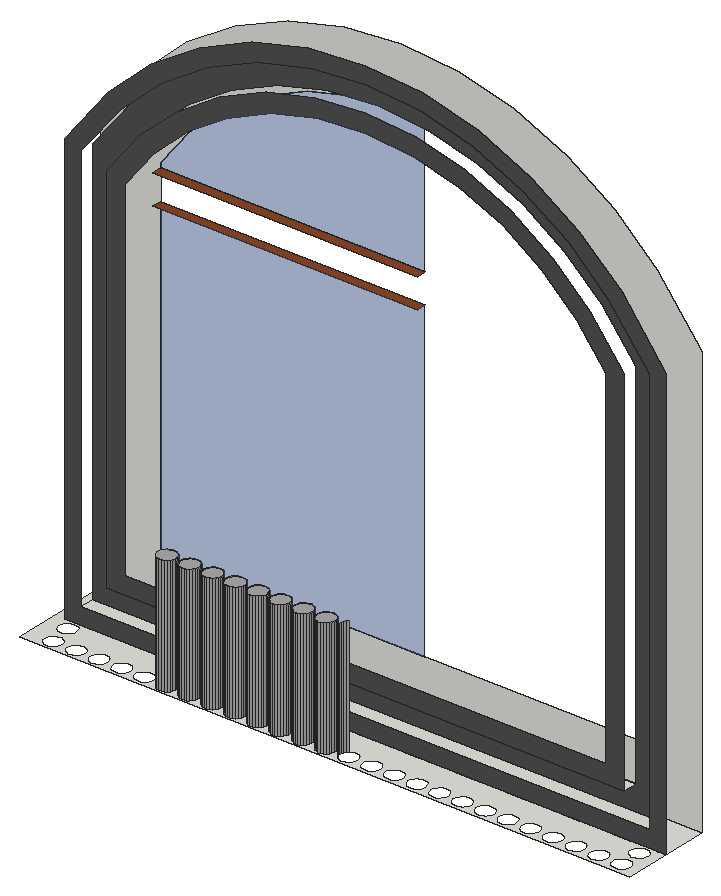
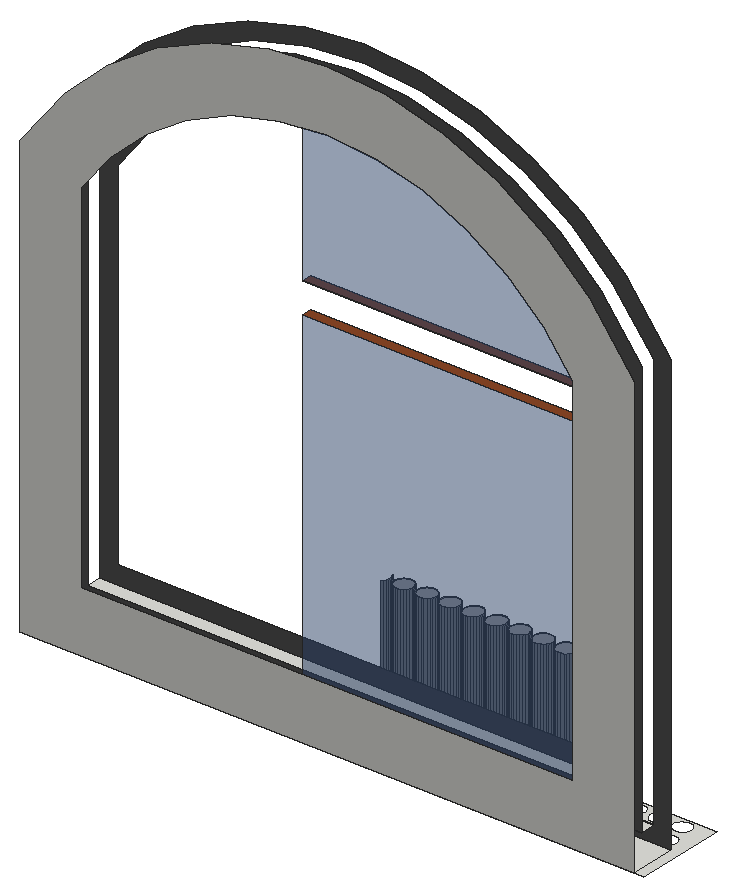
# SketchUp Ruby script. Lengths in inches.
U = 1.inch
M = Sketchup.active_model
def pt(a) = Geom::Point3d.new(a.map { |v| v * U })
def face(e, loops, mat)
  f = e.add_face(loops[0].map { |a| pt(a) })
  loops[1..].each { |l| e.add_face(l.map { |a| pt(a) }).erase! }
  f.material = f.back_material = mat if mat
  f
end
# faces: each face lists its corners as indices into pts; further lists are holes
def faces(e, pts, list, mat = nil) = list.each { |f| face(e, (f[0].is_a?(Array) ? f : [f]).map { |l| l.map { |i| pts[i] } }, mat) }
# xy, xz, yz: faces in a plane at the given z, y or x. An outline is a flat list of corners, or four numbers for a rectangle; further outlines are holes
def ring(l) = l.size == 4 ? [[l[0], l[1]], [l[2], l[1]], [l[2], l[3]], [l[0], l[3]]] : l.each_slice(2).to_a
def flat(e, list, mat, &to3) = list.each { |f| face(e, (f[0].is_a?(Array) ? f : [f]).map { |l| ring(l).map { |u, v| to3.(u, v) } }, mat) }
def xy(e, z, list, mat = nil) = flat(e, list, mat) { |x, y| [x, y, z] }
def xz(e, y, list, mat = nil) = flat(e, list, mat) { |x, z| [x, y, z] }
def yz(e, x, list, mat = nil) = flat(e, list, mat) { |y, z| [x, y, z] }
def lines(e, pts, list) = list.each { |a, b| e.add_line(pt(pts[a]), pt(pts[b])) }
# prism: a flat outline (further loops are holes) pulled along v
def prism(e, loops, v, mat = nil)
  f = face(e, loops, mat); d = Geom::Vector3d.new(v.map { |x| x * U })
  f.pushpull(f.normal.samedirection?(d) ? d.length : -d.length)
end
def box(e, o, s, mat = nil) = prism(e, [[o, [o[0] + s[0], o[1], o[2]], [o[0] + s[0], o[1] + s[1], o[2]], [o[0], o[1] + s[1], o[2]]]], [0, 0, s[2]], mat)
def at(x, y, z, deg = 0) = Geom::Transformation.translation(pt([x, y, z])) * Geom::Transformation.rotation(ORIGIN, Z_AXIS, deg.degrees)
def axes(o, x, y, z) = Geom::Transformation.new([*x, 0, *y, 0, *z, 0, *pt(o).to_a, 1])
def part(name) = M.definitions.add(name)
# library, detail: a bought-in or finely detailed component or shape, given as its bounding box
def library(name, o, s) = part(name).tap { |d| box(d.entities, o, s) }
def detail(e, o, s) = box(e.add_group.entities, o, s)
def put(e, d, t, mat = nil) = e.add_instance(d, t).tap { |i| i.material = mat if mat }
def group(e, t, mat = nil) = e.add_group.tap { |g| g.transformation = t; g.material = mat if mat }.entities
root = M.entities
M.materials.add("[0042_Sienna]").color = [137, 70, 38]
M.materials.add("[0132_LightGray]").color = [169, 169, 169]
M.materials.add("[0135_DarkGray]").color = [81, 81, 81]
M.materials.add("[Translucent Glass Blue]").color = [66, 99, 158]
M.materials["[Translucent Glass Blue]"].alpha = 0.5
xy(root,336.85,[[[238.64,31.6875,361.14,31.6875,361.14,40.6875,240.45,40.6875,240.45,49.6875,238.64,49.6875],[357.52,36.54,357.06,36.64,356.64,36.85,356.29,37.17,356.03,37.57,355.88,38.02,355.86,38.49,355.95,38.95,356.17,39.375,356.48,39.73,356.88,39.98,357.33,40.13,357.8,40.16,358.27,40.06,358.6875,39.84,359.04,39.53,359.3,39.13,359.44,38.68,359.47,38.21,359.37,37.75,359.16,37.32,358.84,36.97,358.44,36.71,357.99,36.57],[242.65,36.72,242.18,36.82,241.76,37.03,241.41,37.35,241.15,37.75,241,38.2,240.98,38.67,241.08,39.13,241.29,39.55,241.61,39.91,242.01,40.16,242.45,40.31,242.93,40.34,243.39,40.24,243.8125,40.02,244.16,39.71,244.42,39.31,244.57,38.86,244.59,38.39,244.5,37.92,244.28,37.5,243.96,37.15,243.57,36.89,243.12,36.75],[243.46,32.1,243,32.2,242.57,32.42,242.22,32.73,241.97,33.13,241.82,33.58,241.79,34.05,241.89,34.52,242.11,34.9375,242.42,35.29,242.82,35.55,243.27,35.69,243.74,35.72,244.2,35.62,244.625,35.41,244.98,35.09,245.24,34.69,245.38,34.24,245.41,33.77,245.31,33.31,245.09,32.89,244.78,32.53,244.38,32.28,243.93,32.13],[248.02,32.1,247.56,32.2,247.14,32.42,246.79,32.73,246.53,33.13,246.38,33.58,246.36,34.05,246.45,34.52,246.67,34.9375,246.98,35.29,247.38,35.55,247.83,35.69,248.3,35.72,248.77,35.62,249.1875,35.41,249.54,35.09,249.8,34.69,249.94,34.24,249.97,33.77,249.87,33.31,249.66,32.89,249.34,32.53,248.94,32.28,248.49,32.13],[252.58,32.1,252.12,32.2,251.7,32.42,251.35,32.73,251.09,33.13,250.94,33.58,250.92,34.05,251.02,34.52,251.23,34.9375,251.55,35.29,251.94,35.55,252.39,35.69,252.87,35.72,253.33,35.62,253.75,35.41,254.1,35.09,254.36,34.69,254.51,34.24,254.53,33.77,254.43,33.31,254.22,32.89,253.9,32.53,253.51,32.28,253.06,32.13],[257.15,32.1,256.68,32.2,256.26,32.42,255.91,32.73,255.65,33.13,255.51,33.58,255.48,34.05,255.58,34.52,255.79,34.9375,256.11,35.29,256.51,35.55,256.96,35.69,257.43,35.72,257.89,35.62,258.3125,35.41,258.67,35.09,258.92,34.69,259.07,34.24,259.09,33.77,259,33.31,258.78,32.89,258.47,32.53,258.07,32.28,257.62,32.13],[261.71,32.1,261.25,32.2,260.82,32.42,260.47,32.73,260.22,33.13,260.07,33.58,260.04,34.05,260.14,34.52,260.36,34.9375,260.67,35.29,261.07,35.55,261.52,35.69,261.99,35.72,262.45,35.62,262.875,35.41,263.23,35.09,263.49,34.69,263.63,34.24,263.66,33.77,263.56,33.31,263.34,32.89,263.03,32.53,262.63,32.28,262.18,32.13],[266.27,32.1,265.81,32.2,265.39,32.42,265.04,32.73,264.78,33.13,264.63,33.58,264.61,34.05,264.7,34.52,264.92,34.9375,265.23,35.29,265.63,35.55,266.08,35.69,266.55,35.72,267.02,35.62,267.4375,35.41,267.79,35.09,268.05,34.69,268.19,34.24,268.22,33.77,268.12,33.31,267.91,32.89,267.59,32.53,267.19,32.28,266.74,32.13],[270.83,32.1,270.37,32.2,269.95,32.42,269.6,32.73,269.34,33.13,269.19,33.58,269.17,34.05,269.27,34.52,269.48,34.9375,269.8,35.29,270.19,35.55,270.64,35.69,271.12,35.72,271.58,35.62,272,35.41,272.35,35.09,272.61,34.69,272.76,34.24,272.78,33.77,272.68,33.31,272.47,32.89,272.15,32.53,271.76,32.28,271.31,32.13],[275.4,32.1,274.93,32.2,274.51,32.42,274.16,32.73,273.9,33.13,273.76,33.58,273.73,34.05,273.83,34.52,274.04,34.9375,274.36,35.29,274.76,35.55,275.21,35.69,275.68,35.72,276.14,35.62,276.5625,35.41,276.92,35.09,277.17,34.69,277.32,34.24,277.34,33.77,277.25,33.31,277.03,32.89,276.72,32.53,276.32,32.28,275.87,32.13],[279.96,32.1,279.5,32.2,279.07,32.42,278.72,32.73,278.47,33.13,278.32,33.58,278.29,34.05,278.39,34.52,278.61,34.9375,278.92,35.29,279.32,35.55,279.77,35.69,280.24,35.72,280.7,35.62,281.125,35.41,281.48,35.09,281.74,34.69,281.88,34.24,281.91,33.77,281.81,33.31,281.59,32.89,281.28,32.53,280.88,32.28,280.43,32.13],[284.52,32.1,284.06,32.2,283.64,32.42,283.29,32.73,283.03,33.13,282.88,33.58,282.86,34.05,282.95,34.52,283.17,34.9375,283.48,35.29,283.88,35.55,284.33,35.69,284.8,35.72,285.27,35.62,285.6875,35.41,286.04,35.09,286.3,34.69,286.44,34.24,286.47,33.77,286.37,33.31,286.16,32.89,285.84,32.53,285.44,32.28,284.99,32.13],[289.08,32.1,288.62,32.2,288.2,32.42,287.85,32.73,287.59,33.13,287.44,33.58,287.42,34.05,287.52,34.52,287.73,34.9375,288.05,35.29,288.44,35.55,288.89,35.69,289.37,35.72,289.83,35.62,290.25,35.41,290.6,35.09,290.86,34.69,291.01,34.24,291.03,33.77,290.93,33.31,290.72,32.89,290.4,32.53,290.01,32.28,289.56,32.13],[293.65,32.1,293.18,32.2,292.76,32.42,292.41,32.73,292.15,33.13,292.01,33.58,291.98,34.05,292.08,34.52,292.29,34.9375,292.61,35.29,293.01,35.55,293.46,35.69,293.93,35.72,294.39,35.62,294.8125,35.41,295.17,35.09,295.42,34.69,295.57,34.24,295.59,33.77,295.5,33.31,295.28,32.89,294.97,32.53,294.57,32.28,294.12,32.13],[298.21,32.1,297.75,32.2,297.32,32.42,296.97,32.73,296.72,33.13,296.57,33.58,296.54,34.05,296.64,34.52,296.86,34.9375,297.17,35.29,297.57,35.55,298.02,35.69,298.49,35.72,298.95,35.62,299.375,35.41,299.73,35.09,299.99,34.69,300.13,34.24,300.16,33.77,300.06,33.31,299.84,32.89,299.53,32.53,299.13,32.28,298.68,32.13],[302.77,32.1,302.31,32.2,301.89,32.42,301.54,32.73,301.28,33.13,301.13,33.58,301.11,34.05,301.2,34.52,301.42,34.9375,301.73,35.29,302.13,35.55,302.58,35.69,303.05,35.72,303.52,35.62,303.9375,35.41,304.29,35.09,304.55,34.69,304.69,34.24,304.72,33.77,304.62,33.31,304.41,32.89,304.09,32.53,303.69,32.28,303.24,32.13],[307.33,32.1,306.87,32.2,306.45,32.42,306.1,32.73,305.84,33.13,305.69,33.58,305.67,34.05,305.77,34.52,305.98,34.9375,306.3,35.29,306.69,35.55,307.14,35.69,307.62,35.72,308.08,35.62,308.5,35.41,308.85,35.09,309.11,34.69,309.26,34.24,309.28,33.77,309.18,33.31,308.97,32.89,308.65,32.53,308.26,32.28,307.81,32.13],[311.9,32.1,311.43,32.2,311.01,32.42,310.66,32.73,310.4,33.13,310.26,33.58,310.23,34.05,310.33,34.52,310.54,34.9375,310.86,35.29,311.26,35.55,311.71,35.69,312.18,35.72,312.64,35.62,313.0625,35.41,313.42,35.09,313.67,34.69,313.82,34.24,313.84,33.77,313.75,33.31,313.53,32.89,313.22,32.53,312.82,32.28,312.37,32.13],[316.46,32.1,316,32.2,315.57,32.42,315.22,32.73,314.97,33.13,314.82,33.58,314.79,34.05,314.89,34.52,315.11,34.9375,315.42,35.29,315.82,35.55,316.27,35.69,316.74,35.72,317.2,35.62,317.625,35.41,317.98,35.09,318.24,34.69,318.38,34.24,318.41,33.77,318.31,33.31,318.09,32.89,317.78,32.53,317.38,32.28,316.93,32.13],[321.02,32.1,320.56,32.2,320.14,32.42,319.79,32.73,319.53,33.13,319.38,33.58,319.36,34.05,319.45,34.52,319.67,34.9375,319.98,35.29,320.38,35.55,320.83,35.69,321.3,35.72,321.77,35.62,322.1875,35.41,322.54,35.09,322.8,34.69,322.94,34.24,322.97,33.77,322.87,33.31,322.66,32.89,322.34,32.53,321.94,32.28,321.49,32.13],[325.58,32.1,325.12,32.2,324.7,32.42,324.35,32.73,324.09,33.13,323.94,33.58,323.92,34.05,324.02,34.52,324.23,34.9375,324.55,35.29,324.94,35.55,325.39,35.69,325.87,35.72,326.33,35.62,326.75,35.41,327.1,35.09,327.36,34.69,327.51,34.24,327.53,33.77,327.43,33.31,327.22,32.89,326.9,32.53,326.51,32.28,326.06,32.13],[330.15,32.1,329.68,32.2,329.26,32.42,328.91,32.73,328.65,33.13,328.51,33.58,328.48,34.05,328.58,34.52,328.79,34.9375,329.11,35.29,329.51,35.55,329.96,35.69,330.43,35.72,330.89,35.62,331.3125,35.41,331.67,35.09,331.92,34.69,332.07,34.24,332.09,33.77,332,33.31,331.78,32.89,331.47,32.53,331.07,32.28,330.62,32.13],[334.71,32.1,334.25,32.2,333.82,32.42,333.47,32.73,333.22,33.13,333.07,33.58,333.04,34.05,333.14,34.52,333.36,34.9375,333.67,35.29,334.07,35.55,334.52,35.69,334.99,35.72,335.45,35.62,335.875,35.41,336.23,35.09,336.49,34.69,336.63,34.24,336.66,33.77,336.56,33.31,336.34,32.89,336.03,32.53,335.63,32.28,335.18,32.13],[339.27,32.1,338.81,32.2,338.39,32.42,338.04,32.73,337.78,33.13,337.63,33.58,337.61,34.05,337.7,34.52,337.92,34.9375,338.23,35.29,338.63,35.55,339.08,35.69,339.55,35.72,340.02,35.62,340.4375,35.41,340.79,35.09,341.05,34.69,341.19,34.24,341.22,33.77,341.12,33.31,340.91,32.89,340.59,32.53,340.19,32.28,339.74,32.13],[343.83,32.1,343.37,32.2,342.95,32.42,342.6,32.73,342.34,33.13,342.19,33.58,342.17,34.05,342.27,34.52,342.48,34.9375,342.8,35.29,343.19,35.55,343.64,35.69,344.12,35.72,344.58,35.62,345,35.41,345.35,35.09,345.61,34.69,345.76,34.24,345.78,33.77,345.68,33.31,345.47,32.89,345.15,32.53,344.76,32.28,344.31,32.13],[348.4,32.1,347.93,32.2,347.51,32.42,347.16,32.73,346.9,33.13,346.76,33.58,346.73,34.05,346.83,34.52,347.04,34.9375,347.36,35.29,347.76,35.55,348.21,35.69,348.68,35.72,349.14,35.62,349.5625,35.41,349.92,35.09,350.17,34.69,350.32,34.24,350.34,33.77,350.25,33.31,350.03,32.89,349.72,32.53,349.32,32.28,348.87,32.13],[352.96,32.1,352.5,32.2,352.07,32.42,351.72,32.73,351.47,33.13,351.32,33.58,351.29,34.05,351.39,34.52,351.61,34.9375,351.92,35.29,352.32,35.55,352.77,35.69,353.24,35.72,353.7,35.62,354.125,35.41,354.48,35.09,354.74,34.69,354.88,34.24,354.91,33.77,354.81,33.31,354.59,32.89,354.28,32.53,353.88,32.28,353.43,32.13],[357.52,32.1,357.06,32.2,356.64,32.42,356.29,32.73,356.03,33.13,355.88,33.58,355.86,34.05,355.95,34.52,356.17,34.9375,356.48,35.29,356.88,35.55,357.33,35.69,357.8,35.72,358.27,35.62,358.6875,35.41,359.04,35.09,359.3,34.69,359.44,34.24,359.47,33.77,359.37,33.31,359.16,32.89,358.84,32.53,358.44,32.28,357.99,32.13]],[266.27,32.1,265.81,32.2,265.39,32.42,265.04,32.73,264.78,33.13,264.63,33.58,264.61,34.05,264.7,34.52,264.92,34.9375,265.23,35.29,265.63,35.55,266.08,35.69,266.55,35.72,267.02,35.62,267.4375,35.41,267.79,35.09,268.05,34.69,268.19,34.24,268.22,33.77,268.12,33.31,267.91,32.89,267.59,32.53,267.19,32.28,266.74,32.13],[270.83,32.1,270.37,32.2,269.95,32.42,269.6,32.73,269.34,33.13,269.19,33.58,269.17,34.05,269.27,34.52,269.48,34.9375,269.8,35.29,270.19,35.55,270.64,35.69,271.12,35.72,271.58,35.62,272,35.41,272.35,35.09,272.61,34.69,272.76,34.24,272.78,33.77,272.68,33.31,272.47,32.89,272.15,32.53,271.76,32.28,271.31,32.13],[275.4,32.1,274.93,32.2,274.51,32.42,274.16,32.73,273.9,33.13,273.76,33.58,273.73,34.05,273.83,34.52,274.04,34.9375,274.36,35.29,274.76,35.55,275.21,35.69,275.68,35.72,276.14,35.62,276.5625,35.41,276.92,35.09,277.17,34.69,277.32,34.24,277.34,33.77,277.25,33.31,277.03,32.89,276.72,32.53,276.32,32.28,275.87,32.13],[279.96,32.1,279.5,32.2,279.07,32.42,278.72,32.73,278.47,33.13,278.32,33.58,278.29,34.05,278.39,34.52,278.61,34.9375,278.92,35.29,279.32,35.55,279.77,35.69,280.24,35.72,280.7,35.62,281.125,35.41,281.48,35.09,281.74,34.69,281.88,34.24,281.91,33.77,281.81,33.31,281.59,32.89,281.28,32.53,280.88,32.28,280.43,32.13],
  [284.52,32.1,284.06,32.2,283.64,32.42,283.29,32.73,283.03,33.13,282.88,33.58,282.86,34.05,282.95,34.52,283.17,34.9375,283.48,35.29,283.88,35.55,284.33,35.69,284.8,35.72,285.27,35.62,285.6875,35.41,286.04,35.09,286.3,34.69,286.44,34.24,286.47,33.77,286.37,33.31,286.16,32.89,285.84,32.53,285.44,32.28,284.99,32.13],[289.08,32.1,288.62,32.2,288.2,32.42,287.85,32.73,287.59,33.13,287.44,33.58,287.42,34.05,287.52,34.52,287.73,34.9375,288.05,35.29,288.44,35.55,288.89,35.69,289.37,35.72,289.83,35.62,290.25,35.41,290.6,35.09,290.86,34.69,291.01,34.24,291.03,33.77,290.93,33.31,290.72,32.89,290.4,32.53,290.01,32.28,289.56,32.13],[293.65,32.1,293.18,32.2,292.76,32.42,292.41,32.73,292.15,33.13,292.01,33.58,291.98,34.05,292.08,34.52,292.29,34.9375,292.61,35.29,293.01,35.55,293.46,35.69,293.93,35.72,294.39,35.62,294.8125,35.41,295.17,35.09,295.42,34.69,295.57,34.24,295.59,33.77,295.5,33.31,295.28,32.89,294.97,32.53,294.57,32.28,294.12,32.13],[298.21,32.1,297.75,32.2,297.32,32.42,296.97,32.73,296.72,33.13,296.57,33.58,296.54,34.05,296.64,34.52,296.86,34.9375,297.17,35.29,297.57,35.55,298.02,35.69,298.49,35.72,298.95,35.62,299.375,35.41,299.73,35.09,299.99,34.69,300.13,34.24,300.16,33.77,300.06,33.31,299.84,32.89,299.53,32.53,299.13,32.28,298.68,32.13],[240.45,40.6875,361.14,49.6875]])
xy(root,340.14,[[243.74,40.6875,357.84,43.6875]])
xy(root,345.3,[[248.9,40.6875,352.68,43.6875]])
xy(root,360.41,[[266.27,32.1,266.74,32.13,267.19,32.28,267.59,32.53,267.91,32.89,268.12,33.31,268.22,33.77,268.19,34.24,268.05,34.69,267.79,35.09,267.4375,35.41,267.02,35.62,266.55,35.72,266.08,35.69,265.63,35.55,265.23,35.29,264.92,34.9375,264.7,34.52,264.61,34.05,264.63,33.58,264.78,33.13,265.04,32.73,265.39,32.42,265.81,32.2],[270.83,32.1,271.31,32.13,271.76,32.28,272.15,32.53,272.47,32.89,272.68,33.31,272.78,33.77,272.76,34.24,272.61,34.69,272.35,35.09,272,35.41,271.58,35.62,271.12,35.72,270.64,35.69,270.19,35.55,269.8,35.29,269.48,34.9375,269.27,34.52,269.17,34.05,269.19,33.58,269.34,33.13,269.6,32.73,269.95,32.42,270.37,32.2],[275.4,32.1,275.87,32.13,276.32,32.28,276.72,32.53,277.03,32.89,277.25,33.31,277.34,33.77,277.32,34.24,277.17,34.69,276.92,35.09,276.5625,35.41,276.14,35.62,275.68,35.72,275.21,35.69,274.76,35.55,274.36,35.29,274.04,34.9375,273.83,34.52,273.73,34.05,273.76,33.58,273.9,33.13,274.16,32.73,274.51,32.42,274.93,32.2],[279.96,32.1,280.43,32.13,280.88,32.28,281.28,32.53,281.59,32.89,281.81,33.31,281.91,33.77,281.88,34.24,281.74,34.69,281.48,35.09,281.125,35.41,280.7,35.62,280.24,35.72,279.77,35.69,279.32,35.55,278.92,35.29,278.61,34.9375,278.39,34.52,278.29,34.05,278.32,33.58,278.47,33.13,278.72,32.73,279.07,32.42,279.5,32.2],[284.52,32.1,284.99,32.13,285.44,32.28,285.84,32.53,286.16,32.89,286.37,33.31,286.47,33.77,286.44,34.24,286.3,34.69,286.04,35.09,285.6875,35.41,285.27,35.62,284.8,35.72,284.33,35.69,283.88,35.55,283.48,35.29,283.17,34.9375,282.95,34.52,282.86,34.05,282.88,33.58,283.03,33.13,283.29,32.73,283.64,32.42,284.06,32.2],
  [289.08,32.1,289.56,32.13,290.01,32.28,290.4,32.53,290.72,32.89,290.93,33.31,291.03,33.77,291.01,34.24,290.86,34.69,290.6,35.09,290.25,35.41,289.83,35.62,289.37,35.72,288.89,35.69,288.44,35.55,288.05,35.29,287.73,34.9375,287.52,34.52,287.42,34.05,287.44,33.58,287.59,33.13,287.85,32.73,288.2,32.42,288.62,32.2],[293.65,32.1,294.12,32.13,294.57,32.28,294.97,32.53,295.28,32.89,295.5,33.31,295.59,33.77,295.57,34.24,295.42,34.69,295.17,35.09,294.8125,35.41,294.39,35.62,293.93,35.72,293.46,35.69,293.01,35.55,292.61,35.29,292.29,34.9375,292.08,34.52,291.98,34.05,292.01,33.58,292.15,33.13,292.41,32.73,292.76,32.42,293.18,32.2],[298.21,32.1,298.68,32.13,299.13,32.28,299.53,32.53,299.84,32.89,300.06,33.31,300.16,33.77,300.13,34.24,299.99,34.69,299.73,35.09,299.375,35.41,298.95,35.62,298.49,35.72,298.02,35.69,297.57,35.55,297.17,35.29,296.86,34.9375,296.64,34.52,296.54,34.05,296.57,33.58,296.72,33.13,296.97,32.73,297.32,32.42,297.75,32.2]],"[0132_LightGray]")
xy(root,412.18,[[252.45,47.6875,305.64,49.6875]],"[0042_Sienna]")
xy(root,418.18,[[252.45,47.6875,305.64,49.6875]],"[0042_Sienna]")
xz(root,40.6875,[[[240.45,336.85,361.14,336.85,361.14,423.26,352.21,434.86,343.74,442.73,334.09,449.09,323.51,453.76,312.3125,456.61,300.79,457.57,289.27,456.61,278.07,453.76,267.5,449.09,257.84,442.73,249.375,434.86,240.45,423.26],[243.74,340.14,243.74,422.14,251.82,432.64,259.88,440.13,269.08,446.1875,279.15,450.64,289.82,453.36,300.79,454.27,311.76,453.36,322.43,450.64,332.51,446.1875,341.7,440.13,349.77,432.64,357.84,422.14,357.84,340.14]],[[248.9,345.3,352.68,345.3,352.68,420.38,345.9375,429.15,338.5,436.06,330.02,441.64,320.74,445.74,310.91,448.25,300.79,449.09,290.68,448.25,280.84,445.74,271.56,441.64,263.08,436.06,255.65,429.15,248.9,420.38],[252.45,348.85,252.45,419.18,258.28,426.75,265.28,433.26,273.26,438.52,282,442.38,291.27,444.74,300.79,445.53,310.32,444.74,319.58,442.38,328.32,438.52,336.3,433.26,343.31,426.75,349.14,419.18,349.14,348.85]]],"[0135_DarkGray]")
xz(root,43.6875,[[[243.74,340.14,357.84,340.14,357.84,422.14,349.77,432.64,341.7,440.13,332.51,446.1875,322.43,450.64,311.76,453.36,300.79,454.27,289.82,453.36,279.15,450.64,269.08,446.1875,259.88,440.13,251.82,432.64,243.74,422.14],[248.9,345.3,248.9,420.38,255.65,429.15,263.08,436.06,271.56,441.64,280.84,445.74,290.68,448.25,300.79,449.09,310.91,448.25,320.74,445.74,330.02,441.64,338.5,436.06,345.9375,429.15,352.68,420.38,352.68,345.3]]],"[0135_DarkGray]")
xz(root,49.6875,[[[240.45,336.85,240.45,423.26,249.375,434.86,257.84,442.73,267.5,449.09,278.07,453.76,289.27,456.61,300.79,457.57,312.3125,456.61,323.51,453.76,334.09,449.09,343.74,442.73,352.21,434.86,361.14,423.26,361.14,336.85],[252.45,348.85,349.14,348.85,349.14,419.18,343.31,426.75,336.3,433.26,328.32,438.52,319.58,442.38,311.64,444.4,310.32,444.74,305.64,445.13,300.79,445.53,291.27,444.74,282,442.38,273.26,438.52,265.28,433.26,258.28,426.75,252.45,419.18]]])
xz(root,49.6875,[[252.45,348.85,305.64,412.18],[252.45,418.18,305.64,418.18,305.64,445.13,300.79,445.53,291.27,444.74,282,442.38,273.26,438.52,265.28,433.26,258.28,426.75,252.45,419.18]],"[Translucent Glass Blue]")
p = [[265.81,32.2,336.85],[266.27,32.1,336.85],[266.27,32.1,360.41],[265.81,32.2,360.41],[266.74,32.13,336.85],[266.74,32.13,360.41],
  [267.19,32.28,336.85],[267.19,32.28,360.41],[270.37,32.2,336.85],[270.83,32.1,336.85],[270.83,32.1,360.41],[270.37,32.2,360.41],
  [271.31,32.13,336.85],[271.31,32.13,360.41],[271.76,32.28,336.85],[271.76,32.28,360.41],[274.93,32.2,336.85],[275.4,32.1,336.85],
  [275.4,32.1,360.41],[274.93,32.2,360.41],[275.87,32.13,336.85],[275.87,32.13,360.41],[276.32,32.28,336.85],[276.32,32.28,360.41],
  [279.5,32.2,336.85],[279.96,32.1,336.85],[279.96,32.1,360.41],[279.5,32.2,360.41],[280.43,32.13,336.85],[280.43,32.13,360.41],
  [280.88,32.28,336.85],[280.88,32.28,360.41],[284.06,32.2,336.85],[284.52,32.1,336.85],[284.52,32.1,360.41],[284.06,32.2,360.41],
  [284.99,32.13,336.85],[284.99,32.13,360.41],[285.44,32.28,336.85],[285.44,32.28,360.41],[288.62,32.2,336.85],[289.08,32.1,336.85],
  [289.08,32.1,360.41],[288.62,32.2,360.41],[289.56,32.13,336.85],[289.56,32.13,360.41],[290.01,32.28,336.85],[290.01,32.28,360.41],
  [293.18,32.2,336.85],[293.65,32.1,336.85],[293.65,32.1,360.41],[293.18,32.2,360.41],[294.12,32.13,336.85],[294.12,32.13,360.41],
  [294.57,32.28,336.85],[294.57,32.28,360.41],[297.75,32.2,336.85],[298.21,32.1,336.85],[298.21,32.1,360.41],[297.75,32.2,360.41],
  [298.68,32.13,336.85],[298.68,32.13,360.41],[299.13,32.28,336.85],[299.13,32.28,360.41],[265.39,32.42,336.85],[265.39,32.42,360.41],
  [269.95,32.42,336.85],[269.95,32.42,360.41],[274.51,32.42,336.85],[274.51,32.42,360.41],[279.07,32.42,336.85],[279.07,32.42,360.41],
  [283.64,32.42,336.85],[283.64,32.42,360.41],[288.2,32.42,336.85],[288.2,32.42,360.41],[292.76,32.42,336.85],[292.76,32.42,360.41],
  [297.32,32.42,336.85],[297.32,32.42,360.41],[267.59,32.53,336.85],[267.59,32.53,360.41],[272.15,32.53,336.85],[272.15,32.53,360.41],
  [276.72,32.53,336.85],[276.72,32.53,360.41],[281.28,32.53,336.85],[281.28,32.53,360.41],[285.84,32.53,336.85],[285.84,32.53,360.41],
  [290.4,32.53,336.85],[290.4,32.53,360.41],[294.97,32.53,336.85],[294.97,32.53,360.41],[299.53,32.53,336.85],[299.53,32.53,360.41],
  [269.6,32.73,336.85],[269.6,32.73,360.41],[274.16,32.73,336.85],[274.16,32.73,360.41],[278.72,32.73,336.85],[278.72,32.73,360.41],
  [283.29,32.73,336.85],[283.29,32.73,360.41],[287.85,32.73,336.85],[287.85,32.73,360.41],[292.41,32.73,336.85],[292.41,32.73,360.41],
  [296.97,32.73,336.85],[296.97,32.73,360.41],[267.91,32.89,336.85],[267.91,32.89,360.41],[272.47,32.89,336.85],[272.47,32.89,360.41],
  [277.03,32.89,336.85],[277.03,32.89,360.41],[281.59,32.89,336.85],[281.59,32.89,360.41],[286.16,32.89,336.85],[286.16,32.89,360.41],
  [290.72,32.89,336.85],[290.72,32.89,360.41],[295.28,32.89,336.85],[295.28,32.89,360.41],[299.84,32.89,336.85],[299.84,32.89,360.41],
  [269.34,33.13,336.85],[269.34,33.13,360.41],[273.9,33.13,336.85],[273.9,33.13,360.41],[278.47,33.13,336.85],[278.47,33.13,360.41],
  [283.03,33.13,336.85],[283.03,33.13,360.41],[287.59,33.13,336.85],[287.59,33.13,360.41],[292.15,33.13,336.85],[292.15,33.13,360.41],
  [296.72,33.13,336.85],[296.72,33.13,360.41],[301.28,33.13,336.85],[301.54,32.73,336.85],[301.54,32.73,360.41],[301.28,33.13,360.41],
  [268.12,33.31,336.85],[268.12,33.31,360.41],[272.68,33.31,336.85],[272.68,33.31,360.41],[277.25,33.31,336.85],[277.25,33.31,360.41],
  [281.81,33.31,336.85],[281.81,33.31,360.41],[286.37,33.31,336.85],[286.37,33.31,360.41],[290.93,33.31,336.85],[290.93,33.31,360.41],
  [295.5,33.31,336.85],[295.5,33.31,360.41],[300.06,33.31,336.85],[300.06,33.31,360.41],[269.19,33.58,336.85],[269.19,33.58,360.41],
  [273.76,33.58,336.85],[273.76,33.58,360.41],[278.32,33.58,336.85],[278.32,33.58,360.41],[282.88,33.58,336.85],[282.88,33.58,360.41],
  [287.44,33.58,336.85],[287.44,33.58,360.41],[292.01,33.58,336.85],[292.01,33.58,360.41],[296.57,33.58,336.85],[296.57,33.58,360.41],
  [301.13,33.58,336.85],[301.13,33.58,360.41],[268.22,33.77,336.85],[268.22,33.77,360.41],[272.78,33.77,336.85],[272.78,33.77,360.41],
  [277.34,33.77,336.85],[277.34,33.77,360.41],[281.91,33.77,336.85],[281.91,33.77,360.41],[286.47,33.77,336.85],[286.47,33.77,360.41],
  [291.03,33.77,336.85],[291.03,33.77,360.41],[295.59,33.77,336.85],[295.59,33.77,360.41],[300.16,33.77,336.85],[300.16,33.77,360.41],
  [269.17,34.05,336.85],[269.17,34.05,360.41],[273.73,34.05,336.85],[273.73,34.05,360.41],[278.29,34.05,336.85],[278.29,34.05,360.41],
  [282.86,34.05,336.85],[282.86,34.05,360.41],[287.42,34.05,336.85],[287.42,34.05,360.41],[291.98,34.05,336.85],[291.98,34.05,360.41],
  [296.54,34.05,336.85],[296.54,34.05,360.41],[301.11,34.05,336.85],[301.11,34.05,360.41],[268.19,34.24,336.85],[268.19,34.24,360.41],
  [272.76,34.24,336.85],[272.76,34.24,360.41],[277.32,34.24,336.85],[277.32,34.24,360.41],[281.88,34.24,336.85],[281.88,34.24,360.41],
  [286.44,34.24,336.85],[286.44,34.24,360.41],[291.01,34.24,336.85],[291.01,34.24,360.41],[295.57,34.24,336.85],[295.57,34.24,360.41],
  [300.13,34.24,336.85],[300.13,34.24,360.41],[269.27,34.52,336.85],[269.27,34.52,360.41],[273.83,34.52,336.85],[273.83,34.52,360.41],
  [278.39,34.52,336.85],[278.39,34.52,360.41],[282.95,34.52,336.85],[282.95,34.52,360.41],[287.52,34.52,336.85],[287.52,34.52,360.41],
  [292.08,34.52,336.85],[292.08,34.52,360.41],[296.64,34.52,336.85],[296.64,34.52,360.41],[301.2,34.52,336.85],[301.2,34.52,360.41],
  [268.05,34.69,336.85],[268.05,34.69,360.41],[272.61,34.69,336.85],[272.61,34.69,360.41],[277.17,34.69,336.85],[277.17,34.69,360.41],
  [281.74,34.69,336.85],[281.74,34.69,360.41],[286.3,34.69,336.85],[286.3,34.69,360.41],[290.86,34.69,336.85],[290.86,34.69,360.41],
  [295.42,34.69,336.85],[295.42,34.69,360.41],[299.99,34.69,336.85],[299.99,34.69,360.41],[269.48,34.9375,336.85],[269.48,34.9375,360.41],
  [274.04,34.9375,336.85],[274.04,34.9375,360.41],[278.61,34.9375,336.85],[278.61,34.9375,360.41],[283.17,34.9375,336.85],[283.17,34.9375,360.41],
  [287.73,34.9375,336.85],[287.73,34.9375,360.41],[292.29,34.9375,336.85],[292.29,34.9375,360.41],[296.86,34.9375,336.85],[296.86,34.9375,360.41],
  [301.42,34.9375,336.85],[301.42,34.9375,360.41],[267.79,35.09,336.85],[267.79,35.09,360.41],[272.35,35.09,336.85],[272.35,35.09,360.41],
  [276.92,35.09,336.85],[276.92,35.09,360.41],[281.48,35.09,336.85],[281.48,35.09,360.41],[286.04,35.09,336.85],[286.04,35.09,360.41],
  [290.6,35.09,336.85],[290.6,35.09,360.41],[295.17,35.09,336.85],[295.17,35.09,360.41],[299.73,35.09,336.85],[299.73,35.09,360.41],
  [269.8,35.29,336.85],[269.8,35.29,360.41],[274.36,35.29,336.85],[274.36,35.29,360.41],[278.92,35.29,336.85],[278.92,35.29,360.41],
  [283.48,35.29,336.85],[283.48,35.29,360.41],[288.05,35.29,336.85],[288.05,35.29,360.41],[292.61,35.29,336.85],[292.61,35.29,360.41],
  [297.17,35.29,336.85],[297.17,35.29,360.41],[301.73,35.29,336.85],[301.73,35.29,360.41],[267.4375,35.41,336.85],[267.4375,35.41,360.41],
  [272,35.41,336.85],[272,35.41,360.41],[276.5625,35.41,336.85],[276.5625,35.41,360.41],[281.125,35.41,336.85],[281.125,35.41,360.41],
  [285.6875,35.41,336.85],[285.6875,35.41,360.41],[290.25,35.41,336.85],[290.25,35.41,360.41],[294.8125,35.41,336.85],[294.8125,35.41,360.41],
  [299.375,35.41,336.85],[299.375,35.41,360.41],[270.19,35.55,336.85],[270.19,35.55,360.41],[274.76,35.55,336.85],[274.76,35.55,360.41],
  [279.32,35.55,336.85],[279.32,35.55,360.41],[283.88,35.55,336.85],[283.88,35.55,360.41],[288.44,35.55,336.85],[288.44,35.55,360.41],
  [293.01,35.55,336.85],[293.01,35.55,360.41],[297.57,35.55,336.85],[297.57,35.55,360.41],[267.02,35.62,336.85],[267.02,35.62,360.41],
  [271.58,35.62,336.85],[271.58,35.62,360.41],[276.14,35.62,336.85],[276.14,35.62,360.41],[280.7,35.62,336.85],[280.7,35.62,360.41],
  [285.27,35.62,336.85],[285.27,35.62,360.41],[289.83,35.62,336.85],[289.83,35.62,360.41],[294.39,35.62,336.85],[294.39,35.62,360.41],
  [298.95,35.62,336.85],[298.95,35.62,360.41],[266.08,35.69,336.85],[265.63,35.55,336.85],[265.63,35.55,360.41],[266.08,35.69,360.41],
  [270.64,35.69,336.85],[270.64,35.69,360.41],[275.21,35.69,336.85],[275.21,35.69,360.41],[279.77,35.69,336.85],[279.77,35.69,360.41],
  [284.33,35.69,336.85],[284.33,35.69,360.41],[288.89,35.69,336.85],[288.89,35.69,360.41],[293.46,35.69,336.85],[293.46,35.69,360.41],
  [298.02,35.69,336.85],[298.02,35.69,360.41],[266.55,35.72,336.85],[266.55,35.72,360.41],[271.12,35.72,336.85],[271.12,35.72,360.41],
  [275.68,35.72,336.85],[275.68,35.72,360.41],[280.24,35.72,336.85],[280.24,35.72,360.41],[284.8,35.72,336.85],[284.8,35.72,360.41],
  [289.37,35.72,336.85],[289.37,35.72,360.41],[293.93,35.72,336.85],[293.93,35.72,360.41],[298.49,35.72,336.85],[298.49,35.72,360.41]]
faces(root,p,[[0,1,2,3],[1,4,5,2],[4,6,7,5],[8,9,10,11],[9,12,13,10],[12,14,15,13],[16,17,18,19],[17,20,21,18],
  [20,22,23,21],[24,25,26,27],[25,28,29,26],[28,30,31,29],[32,33,34,35],[33,36,37,34],[36,38,39,37],[40,41,42,43],
  [41,44,45,42],[44,46,47,45],[48,49,50,51],[49,52,53,50],[52,54,55,53],[56,57,58,59],[57,60,61,58],[60,62,63,61],
  [64,0,3,65],[66,8,11,67],[68,16,19,69],[70,24,27,71],[72,32,35,73],[74,40,43,75],[76,48,51,77],[78,56,59,79],
  [6,80,81,7],[14,82,83,15],[22,84,85,23],[30,86,87,31],[38,88,89,39],[46,90,91,47],[54,92,93,55],[62,94,95,63],
  [96,66,67,97],[98,68,69,99],[100,70,71,101],[102,72,73,103],[104,74,75,105],[106,76,77,107],[108,78,79,109],[80,110,111,81],
  [82,112,113,83],[84,114,115,85],[86,116,117,87],[88,118,119,89],[90,120,121,91],[92,122,123,93],[94,124,125,95],[126,96,97,127],
  [128,98,99,129],[130,100,101,131],[132,102,103,133],[134,104,105,135],[136,106,107,137],[138,108,109,139],[140,141,142,143],[110,144,145,111],
  [112,146,147,113],[114,148,149,115],[116,150,151,117],[118,152,153,119],[120,154,155,121],[122,156,157,123],[124,158,159,125],[160,126,127,161],
  [162,128,129,163],[164,130,131,165],[166,132,133,167],[168,134,135,169],[170,136,137,171],[172,138,139,173],[174,140,143,175],[144,176,177,145],
  [146,178,179,147],[148,180,181,149],[150,182,183,151],[152,184,185,153],[154,186,187,155],[156,188,189,157],[158,190,191,159],[192,160,161,193],
  [194,162,163,195],[196,164,165,197],[198,166,167,199],[200,168,169,201],[202,170,171,203],[204,172,173,205],[206,174,175,207],[176,208,209,177],
  [178,210,211,179],[180,212,213,181],[182,214,215,183],[184,216,217,185],[186,218,219,187],[188,220,221,189],[190,222,223,191],[224,192,193,225],
  [226,194,195,227],[228,196,197,229],[230,198,199,231],[232,200,201,233],[234,202,203,235],[236,204,205,237],[238,206,207,239],[208,240,241,209],
  [210,242,243,211],[212,244,245,213],[214,246,247,215],[216,248,249,217],[218,250,251,219],[220,252,253,221],[222,254,255,223],[256,224,225,257],
  [258,226,227,259],[260,228,229,261],[262,230,231,263],[264,232,233,265],[266,234,235,267],[268,236,237,269],[270,238,239,271],[240,272,273,241],
  [242,274,275,243],[244,276,277,245],[246,278,279,247],[248,280,281,249],[250,282,283,251],[252,284,285,253],[254,286,287,255],[288,256,257,289],
  [290,258,259,291],[292,260,261,293],[294,262,263,295],[296,264,265,297],[298,266,267,299],[300,268,269,301],[302,270,271,303],[272,304,305,273],
  [274,306,307,275],[276,308,309,277],[278,310,311,279],[280,312,313,281],[282,314,315,283],[284,316,317,285],[286,318,319,287],[320,288,289,321],
  [322,290,291,323],[324,292,293,325],[326,294,295,327],[328,296,297,329],[330,298,299,331],[332,300,301,333],[304,334,335,305],[306,336,337,307],
  [308,338,339,309],[310,340,341,311],[312,342,343,313],[314,344,345,315],[316,346,347,317],[318,348,349,319],[350,351,352,353],[354,320,321,355],
  [356,322,323,357],[358,324,325,359],[360,326,327,361],[362,328,329,363],[364,330,331,365],[366,332,333,367],[334,368,369,335],[336,370,371,337],
  [338,372,373,339],[340,374,375,341],[342,376,377,343],[344,378,379,345],[346,380,381,347],[348,382,383,349],[368,350,353,369],[370,354,355,371],
  [372,356,357,373],[374,358,359,375],[376,360,361,377],[378,362,363,379],[380,364,365,381],[382,366,367,383]],"[0132_LightGray]")
